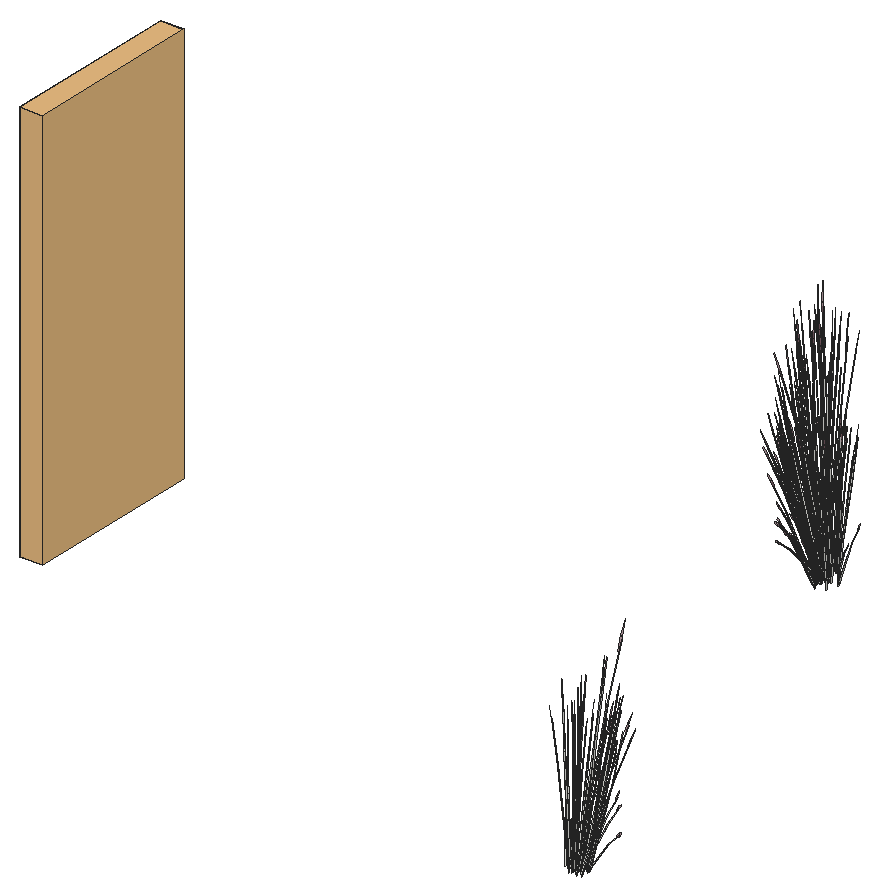
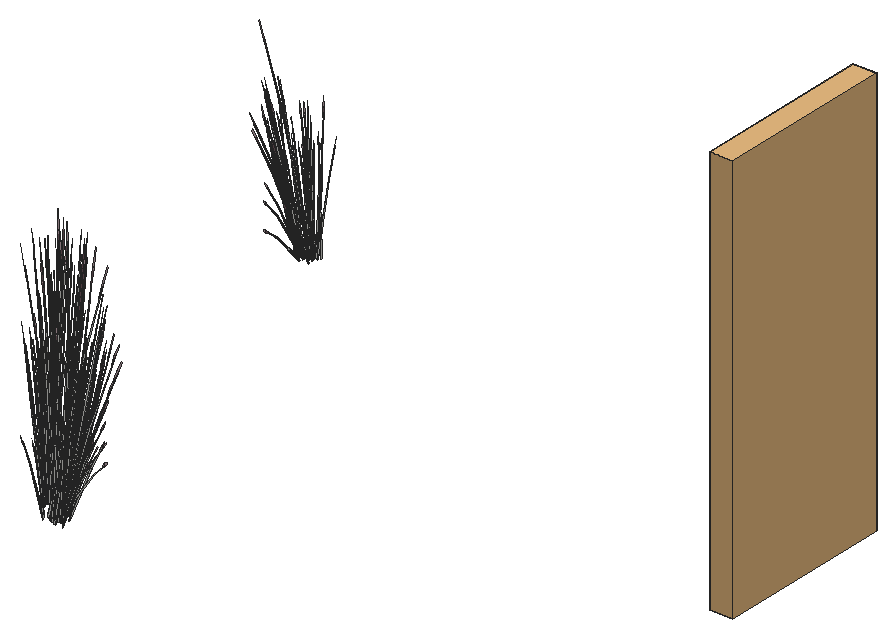
# SketchUp Ruby script. Lengths in inches.
U = 1.inch
M = Sketchup.active_model
def pt(a) = Geom::Point3d.new(a.map { |v| v * U })
def face(e, loops, mat)
  f = e.add_face(loops[0].map { |a| pt(a) })
  loops[1..].each { |l| e.add_face(l.map { |a| pt(a) }).erase! }
  f.material = f.back_material = mat if mat
  f
end
# faces: each face lists its corners as indices into pts; further lists are holes
def faces(e, pts, list, mat = nil) = list.each { |f| face(e, (f[0].is_a?(Array) ? f : [f]).map { |l| l.map { |i| pts[i] } }, mat) }
# xy, xz, yz: faces in a plane at the given z, y or x. An outline is a flat list of corners, or four numbers for a rectangle; further outlines are holes
def ring(l) = l.size == 4 ? [[l[0], l[1]], [l[2], l[1]], [l[2], l[3]], [l[0], l[3]]] : l.each_slice(2).to_a
def flat(e, list, mat, &to3) = list.each { |f| face(e, (f[0].is_a?(Array) ? f : [f]).map { |l| ring(l).map { |u, v| to3.(u, v) } }, mat) }
def xy(e, z, list, mat = nil) = flat(e, list, mat) { |x, y| [x, y, z] }
def xz(e, y, list, mat = nil) = flat(e, list, mat) { |x, z| [x, y, z] }
def yz(e, x, list, mat = nil) = flat(e, list, mat) { |y, z| [x, y, z] }
def lines(e, pts, list) = list.each { |a, b| e.add_line(pt(pts[a]), pt(pts[b])) }
# prism: a flat outline (further loops are holes) pulled along v
def prism(e, loops, v, mat = nil)
  f = face(e, loops, mat); d = Geom::Vector3d.new(v.map { |x| x * U })
  f.pushpull(f.normal.samedirection?(d) ? d.length : -d.length)
end
def box(e, o, s, mat = nil) = prism(e, [[o, [o[0] + s[0], o[1], o[2]], [o[0] + s[0], o[1] + s[1], o[2]], [o[0], o[1] + s[1], o[2]]]], [0, 0, s[2]], mat)
def at(x, y, z, deg = 0) = Geom::Transformation.translation(pt([x, y, z])) * Geom::Transformation.rotation(ORIGIN, Z_AXIS, deg.degrees)
def axes(o, x, y, z) = Geom::Transformation.new([*x, 0, *y, 0, *z, 0, *pt(o).to_a, 1])
def part(name) = M.definitions.add(name)
# library, detail: a bought-in or finely detailed component or shape, given as its bounding box
def library(name, o, s) = part(name).tap { |d| box(d.entities, o, s) }
def detail(e, o, s) = box(e.add_group.entities, o, s)
def put(e, d, t, mat = nil) = e.add_instance(d, t).tap { |i| i.material = mat if mat }
def group(e, t, mat = nil) = e.add_group.tap { |g| g.transformation = t; g.material = mat if mat }.entities
root = M.entities
M.materials.add("LightPink_Translucent").color = [144, 107, 117]
M.materials["LightPink_Translucent"].alpha = 0.75
c1 = part("blade")
p = [[2.15,0.21,22],[0,0.17,0],[0.09,0.45,0],[2.18,0.31,22],[2.29,0.31,22],[0.38,0.45,0],
  [2.48,0.24,33],[2.49,0.24,33],[2.48,0.22,33]]
faces(c1.entities,p,[[0,1,2,3],[4,5,2,3],[6,3,4,7],[8,0,3,6]])
c2 = part("seeds")
p = [[0.3,-0.1,1.38],[-0.01,-0.03,1.59],[-0.01,-0.03,0.03],[0.14,-0.07,-0.07],[0.29,-0.03,3],[0.15,0.01,3.11]]
faces(c2.entities,p,[[0,1,2,3],[1,0,4,5]],"LightPink_Translucent")
c3 = part("blade with seeds")
put(c3.entities,c1,at(0,0,0))
put(c3.entities,c2,axes([2.4,0.25,30.99],[1.5799,-0.05474,1.17369],[-0.12525,1.92788,0.29478],[-0.07173,-0.02425,1.56792]))
c4 = library("porta+4",[0.2,-5.42,1.33],[46.55,4.72,83.21])
put(root,c3,axes([434.05,211.68,2.05],[0.08072,-0.00933,1.50452],[0.22141,-0.42869,-0.23794],[0.14358,0.05659,0.12066]))
put(root,c3,axes([430.82,211.26,2.07],[-0.09332,-0.50785,0.41282],[0.36608,-0.08814,0.34039],[-0.10789,0.11944,0.85423]))
put(root,c3,axes([430.75,211.16,2.07],[-0.25832,-0.23207,0.0553],[0.1504,-0.33047,0.43534],[-0.08282,0.10684,0.66383]))
put(root,c3,axes([430.87,210.55,1.33],[0.13056,-0.11672,1.47384],[0.10992,0.53933,0.11917],[-0.20497,0.12189,0.63005]))
put(root,c3,axes([431.05,211.09,2.34],[0.32754,-0.07886,0.30456],[0.08649,0.45081,-0.39319],[-0.09386,0.12109,0.75234]))
put(root,c3,axes([429.79,210.89,2.05],[0.04802,0.0148,1.5255],[0.14856,0.48754,-0.14414],[-0.0983,0.12796,0.26996]))
put(root,c3,axes([433.97,211.98,1.89],[0.2141,0.34548,-0.30456],[-0.24447,0.32704,0.39319],[0.12421,0.04976,0.75234]))
put(root,c3,axes([433.86,212.11,2.07],[-0.01895,0.4196,0.0553],[-0.28611,-0.0115,0.43534],[0.1096,0.04391,0.66383]))
put(root,c3,axes([430.78,211.36,1.89],[-0.32754,0.07886,-0.30456],[-0.08649,-0.45081,0.39319],[-0.09386,0.12109,0.75234]))
put(root,c3,axes([433.88,211.98,2.07],[-0.27746,0.36359,0.41282],[-0.23929,-0.38612,0.34039],[0.13017,0.06707,0.85423]))
put(root,c3,axes([430.31,212.37,2.86],[0.33205,0.14729,-0.05579],[-0.10214,0.45334,-0.25298],[-0.05431,0.06883,0.83441]))
put(root,c3,axes([433,212.4,2.34],[-0.05812,-0.44446,0.30456],[0.33222,-0.11736,-0.39319],[0.08923,0.12737,0.75234]))
put(root,c3,axes([433.2,211.09,1.33],[-0.13977,-0.09507,1.47384],[0.28925,-0.39884,0.11917],[0.18028,0.17992,0.63005]))
put(root,c3,axes([433.22,209.84,1.85],[-0.32515,-0.2867,1.18923],[0.34333,-0.44639,0.51312],[0.10491,0.26901,1.1495]))
put(root,c3,axes([430.88,211.05,2.33],[0.34807,0.30426,-0.10458],[-0.20053,0.44063,-0.58045],[-0.09834,0.15317,0.88199]))
put(root,c3,axes([432.97,212.625,2.33],[0.22423,-0.47232,-0.10458],[0.32472,0.27211,-0.58045],[0.11288,0.13344,0.88199]))
put(root,c3,axes([431.35,210.91,1.33],[0.09398,-0.16955,1.47384],[0.23731,0.45764,0.11917],[-0.16276,0.20841,0.63005]))
put(root,c3,axes([431.49,211.99,2.34],[0.2546,-0.29052,0.30456],[0.24101,0.33173,-0.39319],[-0.03667,0.16855,0.75234]))
put(root,c3,axes([432.68,213.02,2.05],[0.00111,-0.06681,1.5255],[0.32247,-0.29474,-0.14414],[0.11201,0.1052,0.26996]))
put(root,c3,axes([431.26,212.25,2.07],[-0.30922,-0.02571,0.0553],[0.00848,-0.38824,0.43534],[-0.03236,0.14872,0.66383]))
put(root,c3,axes([431.36,212.29,2.07],[-0.26795,-0.37649,0.41282],[0.28456,-0.3247,0.34039],[-0.04943,0.17664,0.85423]))
put(root,c3,axes([432.21,212.47,2.34],[0.11344,-0.42434,0.30456],[0.33096,0.12377,-0.39319],[0.03035,0.17085,0.75234]))
put(root,c3,axes([433.05,212.8,2.07],[-0.17102,0.35053,0.0553],[-0.24354,-0.20408,0.43534],[0.07874,0.11238,0.66383]))
put(root,c3,axes([432.65,213.98,2.86],[0.26003,-0.31656,-0.05579],[0.23826,0.3467,-0.25298],[0.01677,0.09824,0.83441]))
put(root,c3,axes([433.125,212.7,2.07],[-0.37426,0.12663,0.41282],[-0.06495,-0.49674,0.34039],[0.08802,0.1464,0.85423]))
put(root,c3,axes([431.28,211.33,1.33],[0.07006,-0.18966,1.47384],[0.29392,0.3925,0.11917],[-0.13259,0.24463,0.63005]))
put(root,c3,axes([432.1,212.85,2.07],[-0.27727,0.18753,0.0553],[-0.13571,-0.34197,0.43534],[0.02678,0.15075,0.66383]))
put(root,c3,axes([431.36,212.4,1.89],[-0.2546,0.29052,-0.30456],[-0.24101,-0.33173,0.39319],[-0.03667,0.16855,0.75234]))
put(root,c3,axes([430.48,212.32,2.05],[-0.00935,0.1092,1.50452],[0.26544,0.37987,-0.23794],[-0.06949,0.17964,0.12066]))
put(root,c3,axes([431.33,212.07,2.64],[0.41355,0.02734,-0.11608],[-0.0113,0.51765,-0.6443],[-0.02873,0.19937,0.97901]))
put(root,c3,axes([432.09,212.65,2.33],[0.36822,-0.25691,-0.10458],[0.18095,0.45596,-0.58045],[0.04858,0.19215,0.88199]))
put(root,c3,axes([432.2,212.82,2.35],[-0.37078,-0.14426,0.45823],[0.12679,-0.47426,0.37783],[0.02228,0.18651,0.9482]))
put(root,c3,axes([432.62,211.64,1.33],[-0.08601,-0.17716,1.47384],[0.39746,-0.14915,0.11917],[0.08983,0.27813,0.63005]))
put(root,c3,axes([432.24,212.91,1.89],[-0.11344,0.42434,-0.30456],[-0.33096,-0.12377,0.39319],[0.03035,0.17085,0.75234]))
put(root,c3,axes([430.45,213.43,2.05],[0.04269,-0.03331,1.5255],[0.35284,0.2216,-0.14414],[-0.00829,0.1845,0.26996]))
put(root,c3,axes([431.92,211.73,1.33],[-0.00921,-0.21179,1.47384],[0.39917,0.1405,0.11917],[-0.02469,0.30182,0.63005]))
put(root,c3,axes([432.01,213.67,2.05],[0.0477,0.08886,1.50452],[0.38493,0.03491,-0.23794],[0.03871,0.19596,0.12066]))
put(root,c4,axes([307.84,266.46,4.63],[0,-0.77596,0],[1,0,0],[0,0,0.99642]))
put(root,c3,axes([406.2,304.97,6.33],[0.08601,0.17716,1.47384],[-0.39746,0.14915,0.11917],[-0.08983,-0.27813,0.63005]))
put(root,c3,axes([406.86,303.79,7.05],[-0.05755,-0.07737,1.50452],[-0.38409,0.04905,-0.23794],[-0.0613,-0.18505,0.12066]))
put(root,c3,axes([407.75,304.71,5.23],[-0.10696,0.11169,1.22981],[-0.32033,-0.19549,-0.26449],[0.05938,-0.24312,0.52581]))
put(root,c3,axes([407.26,305.1,7.28],[-0.17959,-0.44867,-0.61099],[0.36969,-0.25004,0.07373],[-0.042,-0.21679,0.8643]))
put(root,c3,axes([406.09,304.5,5.23],[-0.02279,0.18051,1.22981],[-0.33311,0.15111,-0.26449],[-0.07787,-0.23331,0.52581]))
put(root,c3,axes([406.95,304.1,4.28],[-0.06312,0.01988,1.51654],[-0.34903,-0.22379,-0.23168],[0.00586,-0.18666,0.25832]))
put(root,c3,axes([408.01,305.54,7.28],[0.00979,-0.51041,-0.61099],[0.4123,0.03428,0.07373],[0.04351,-0.21623,0.8643]))
put(root,c3,axes([408.58,304.74,7.05],[-0.00363,-0.10982,1.50452],[-0.30678,-0.3174,-0.23794],[0.04743,-0.1924,0.12066]))
put(root,c3,axes([407.29,304.72,6.89],[0.11344,-0.42434,-0.30456],[0.33096,0.12377,0.39319],[-0.03035,-0.17085,0.75234]))
put(root,c3,axes([407.54,305.28,6.33],[-0.07006,0.18966,1.47384],[-0.29392,-0.3925,0.11917],[0.13259,-0.24463,0.63005]))
put(root,c3,axes([408.5,304.35,7.05],[-0.03821,0.04215,1.5255],[-0.37441,-0.1422,-0.14414],[-0.01355,-0.18393,0.26996]))
put(root,c3,axes([407.125,305.01,7.03],[-0.3699,-0.13833,-0.43945],[0.12679,-0.47426,-0.34039],[-0.03392,-0.19095,0.84085]))
put(root,c3,axes([407.35,303.82,5.38],[0.04827,0.32177,0.9878],[-0.26778,-0.17821,0.72577],[0.02882,-0.16476,0.21757]))
put(root,c3,axes([407.92,305.37,7.03],[-0.26937,-0.37076,-0.43945],[0.28456,-0.3247,-0.34039],[0.04099,-0.18838,0.84085]))
put(root,c3,axes([406.46,303.54,7.05],[-0.00702,0.06614,1.5255],[-0.34622,0.24004,-0.14414],[-0.10188,-0.1227,0.26996]))
put(root,c3,axes([406.39,304.71,7.38],[0.41917,-0.14183,0.46236],[0.07275,0.55635,0.38124],[-0.09858,-0.16397,0.95674]))
put(root,c3,axes([407.34,304.82,7.07],[0.37078,0.14426,0.41282],[-0.12679,0.47426,0.34039],[-0.02228,-0.18651,0.85423]))
put(root,c3,axes([407.44,304.99,7.33],[-0.36822,0.25691,-0.10458],[-0.18095,-0.45596,-0.58045],[-0.04858,-0.19215,0.88199]))
put(root,c3,axes([408.21,305.5625,7.33],[-0.41355,-0.02734,-0.10458],[0.0113,-0.51765,-0.58045],[0.02873,-0.19937,0.88199]))
put(root,c3,axes([408.18,305.23,6.89],[0.2546,-0.29052,-0.30456],[0.24101,0.33173,0.39319],[0.03667,-0.16855,0.75234]))
put(root,c3,axes([405.98,304.21,5.38],[0.19628,0.19205,0.9878],[-0.28586,0.11545,0.72577],[-0.06116,-0.1476,0.21757]))
put(root,c3,axes([407.43,304.78,7.07],[0.27727,-0.18753,0.0553],[0.13571,0.34197,0.43534],[-0.02678,-0.15075,0.66383]))
put(root,c3,axes([406.45,305.23,7.28],[-0.32086,-0.26671,-0.61099],[0.22803,-0.46737,0.07373],[-0.11625,-0.15925,0.8643]))
put(root,c3,axes([406.34,304.875,6.89],[-0.05812,-0.44446,-0.30456],[0.33222,-0.11736,0.39319],[-0.08923,-0.12737,0.75234]))
put(root,c3,axes([406.48,304.83,7.07],[0.17102,-0.35053,0.0553],[0.24354,0.20408,0.43534],[-0.07874,-0.11238,0.66383]))
put(root,c3,axes([405.82,304.79,4.28],[-0.03645,0.07269,1.51654],[-0.36835,0.15672,-0.23168],[-0.08898,-0.14257,0.25832]))
put(root,c3,axes([406.43,306.79,4.8],[-0.15453,-0.56584,-0.60058],[0.44514,-0.20379,-0.15763],[-0.01708,-0.19161,1.32568]))
put(root,c3,axes([405.625,305.52,6.33],[0.13977,0.09507,1.47384],[-0.28925,0.39884,0.11917],[-0.18028,-0.17992,0.63005]))
put(root,c3,axes([408.5,305.06,4.28],[-0.05632,-0.04347,1.51654],[-0.14467,-0.48565,-0.23168],[0.09759,-0.13179,0.25832]))
put(root,c3,axes([407.33,305.17,7.34],[-0.11344,0.42434,0.30456],[-0.33096,-0.12377,-0.39319],[-0.03035,-0.17085,0.75234]))
put(root,c3,axes([406.3,305.24,7.03],[-0.37131,0.13117,-0.43945],[-0.06495,-0.49674,-0.34039],[-0.09973,-0.14235,0.84085]))
put(root,c3,axes([408.18,305.34,7.07],[0.26795,0.37649,0.41282],[-0.28456,0.3247,0.34039],[0.04943,-0.17664,0.85423]))
put(root,c3,axes([406.5625,304.8,7.67],[-0.25113,0.52899,-0.11713],[-0.36369,-0.30476,-0.65011],[-0.12642,-0.14945,0.98783]))
put(root,c3,axes([408.28,305.38,7.07],[0.30922,0.02571,0.0553],[-0.00848,0.38824,0.43534],[0.03236,-0.14872,0.66383]))
put(root,c3,axes([408.04,305.64,7.34],[-0.2546,0.29052,0.30456],[-0.24101,-0.33173,-0.39319],[0.03667,-0.16855,0.75234]))
put(root,c3,axes([408.49,306.43,7.28],[0.19655,-0.43539,-0.61099],[0.34443,0.30942,0.07373],[0.11736,-0.15774,0.8643]))
put(root,c3,axes([406.37,305.16,5.04],[-0.23526,-0.55293,0],[0.3936,-0.30836,-0.44382],[0.08964,-0.07023,1.40792]))
put(root,c3,axes([408.48,306.22,7.03],[-0.09666,-0.50384,-0.43945],[0.36608,-0.08814,-0.34039],[0.10491,-0.13533,0.84085]))
put(root,c3,axes([406.89,304.49,4.83],[-0.26003,0.31656,-0.03348],[-0.23826,-0.3467,-0.15179],[-0.01677,-0.09824,0.50065]))
put(root,c3,axes([405.6,304.64,7.05],[-0.08096,-0.00389,1.50452],[-0.25776,0.38949,-0.23794],[-0.13753,-0.07958,0.12066]))
put(root,c3,axes([408.66,306.58,7.33],[-0.34807,-0.30426,-0.10458],[0.20053,-0.44063,-0.58045],[0.09834,-0.15317,0.88199]))
put(root,c3,axes([407.22,308.24,5.86],[0.32517,0.22251,1.30084],[-0.31856,0.47936,0.51441],[-0.14269,-0.28411,1.09053]))
put(root,c3,axes([406.54,305.24,7.34],[0.05812,0.44446,0.30456],[-0.33222,0.11736,-0.39319],[-0.08923,-0.12737,0.75234]))
put(root,c3,axes([405.52,306.71,4.74],[0,-0.5518,-0.427],[0.42099,0,0],[0,-0.12568,1.35453]))
put(root,c3,axes([406.6875,305.07,4.74],[0.35217,-0.2759,-0.427],[0.2105,0.49473,0],[0.08021,-0.06284,1.35453]))
put(root,c3,axes([408.78,306.03,5.23],[-0.13443,-0.01634,1.22981],[-0.13772,-0.43844,-0.26449],[0.16514,-0.12403,0.52581]))
put(root,c3,axes([405.54,305.53,7.38],[0.31075,-0.40722,0.46236],[0.268,0.43246,0.38124],[-0.14579,-0.07512,0.95674]))
put(root,c3,axes([409.51,306.45,7.05],[-0.04915,-0.00419,1.5255],[-0.20409,-0.44904,-0.14414],[0.08196,-0.14765,0.26996]))
put(root,c3,axes([407.11,306.2,4.77],[0.25345,-0.41475,-0.53624],[0.31485,0.37608,-0.14074],[0.10156,-0.10346,1.18365]))
put(root,c3,axes([408.93,305.22,5.38],[-0.12533,0.28089,0.9878],[-0.10773,-0.37739,0.72577],[0.10352,-0.09457,0.21757]))
put(root,c3,axes([408.75,306.28,6.89],[0.32754,-0.07886,-0.30456],[0.08649,0.45081,0.39319],[0.09386,-0.12109,0.75234]))
put(root,c3,axes([405.68,305.52,7.07],[0.01895,-0.4196,0.0553],[0.28611,0.0115,0.43534],[-0.1096,-0.04391,0.66383]))
put(root,c3,axes([406.66,306.93,4.9],[0.18257,-0.49721,-0.38476],[0.37935,0.23929,0.18517],[0,-0.11462,1.23533]))
put(root,c3,axes([405.57,305.66,6.89],[-0.2141,-0.34548,-0.30456],[0.24447,-0.32704,0.39319],[-0.12421,-0.04976,0.75234]))
put(root,c3,axes([406.83,306.69,5.29],[-0.04385,-0.62963,-0.25022],[0.45669,-0.03807,-0.43002],[0.08042,-0.08387,1.37348]))
put(root,c3,axes([405.7,306.72,4.74],[0.26266,-0.34428,-0.26641],[0.26266,0.34428,0.26641],[0,-0.11089,1.19518]))
put(root,c3,axes([405.59,305.07,4.83],[-0.10855,0.45057,-0.03348],[-0.33409,-0.1386,-0.15179],[-0.05073,-0.0737,0.50065]))
put(root,c3,axes([408.49,306.54,7.34],[-0.32754,0.07886,0.30456],[-0.08649,-0.45081,-0.39319],[0.09386,-0.12109,0.75234]))
put(root,c3,axes([406.62,307.34,5.29],[-0.42377,-0.26329,-0.25022],[0.20405,-0.55571,-0.43002],[-0.01332,-0.13644,1.37348]))
put(root,c3,axes([405.41,307.125,5.04],[-0.47052,0,0],[0,-0.61671,-0.44382],[0,-0.14046,1.40792]))
put(root,c3,axes([405.49,306.02,5.23],[0.07347,0.15363,1.22981],[-0.16929,0.41759,-0.26449],[-0.17383,-0.09981,0.52581]))
put(root,c3,axes([406.77,305.29,4.74],[0.35106,0.13653,-0.26641],[-0.08839,0.48081,0.26641],[0.07077,-0.05545,1.19518]))
put(root,c3,axes([405.8,305.89,7.28],[-0.37615,-0.01329,-0.61099],[0.02526,-0.55946,0.07373],[-0.15935,-0.05904,0.8643]))
put(root,c3,axes([408.78,306.47,7.07],[0.25832,0.23207,0.0553],[-0.1504,0.33047,0.43534],[0.08282,-0.10684,0.66383]))
put(root,c3,axes([408.71,306.375,7.07],[0.09332,0.50785,0.41282],[-0.36608,0.08814,0.34039],[0.10789,-0.11944,0.85423]))
put(root,c3,axes([409.7,306.99,7.05],[0.05222,-0.08405,1.50452],[-0.06683,-0.51557,-0.23794],[0.13101,-0.09775,0.12066]))
put(root,c3,axes([405.78,306.96,5],[-0.35001,0.46392,0.2645],[-0.35022,-0.45904,-0.31383],[-0.01222,-0.13174,1.41801]))
put(root,c3,axes([405.29,304.98,7.05],[0.0279,0.05507,1.5255],[-0.13448,0.49501,-0.14414],[-0.1362,0.00358,0.26996]))
put(root,c3,axes([406.89,307.18,5.09],[0.42398,0.26744,0.20696],[-0.20405,0.55571,0.43002],[0,-0.1281,1.38067]))
put(root,c3,axes([406.73,307.93,5.1],[0.09973,-0.65385,-0.20149],[0.47288,0.11397,0.44093],[-0.08263,-0.0903,1.34539]))
put(root,c3,axes([405.67,306,7.03],[-0.27323,0.36552,-0.43945],[-0.23929,-0.38612,-0.34039],[-0.13882,-0.05561,0.84085]))
put(root,c3,axes([405.875,305.84,7.34],[0.2141,0.34548,0.30456],[-0.24447,0.32704,-0.39319],[-0.12421,-0.04976,0.75234]))
put(root,c3,axes([405.06,306.48,5.38],[0.24023,-0.03948,0.9878],[-0.15239,0.3479,0.72577],[-0.11872,-0.05219,0.21757]))
put(root,c3,axes([406.75,306.81,5.34],[-0.40861,0.03406,0.38476],[-0.03695,-0.56543,-0.18517],[0.07315,-0.05731,1.23533]))
put(root,c3,axes([405.82,305.62,7.33],[-0.02015,0.56117,-0.10458],[-0.38148,-0.01534,-0.58045],[-0.14692,-0.03898,0.88199]))
put(root,c3,axes([405.7,307.22,5.13],[0,0.5518,0.427],[-0.42099,0,0],[0,-0.12568,1.35453]))
put(root,c3,axes([408.67,307.77,7.33],[-0.18933,-0.49965,-0.10458],[0.33602,-0.24554,-0.58045],[0.1416,-0.06592,0.88199]))
put(root,c3,axes([408.65,307.34,7.03],[0.10194,-0.50193,-0.43945],[0.34951,0.17204,-0.34039],[0.14072,-0.04602,0.84085]))
put(root,c3,axes([408.1,305.3,5.04],[0.23526,-0.55293,0],[0.3936,0.30836,-0.44382],[0.08964,0.07023,1.40792]))
put(root,c3,axes([405.33,306.39,6.33],[0.15608,-0.0125,1.47384],[-0.10354,0.54165,0.11917],[-0.22242,-0.0335,0.63005]))
put(root,c3,axes([406.69,307.66,4.9],[-0.22605,-0.46315,-0.38476],[0.34239,-0.32614,0.18517],[-0.07315,-0.05731,1.23533]))
put(root,c3,axes([406.74,307.01,5.03],[0.1636,0.61702,0.39349],[-0.46745,0.21456,0.15441],[0.00571,-0.11338,1.36617]))
put(root,c3,axes([409.03,307.48,4.7],[-0.24235,0.06622,1.21762],[-0.03858,-0.5271,0.0697],[0.16974,-0.07978,0.69287]))
put(root,c3,axes([409.47,307.02,4.94],[-0.23329,-0.35284,-0.05579],[0.2555,-0.3233,-0.25298],[0.0724,-0.02276,0.83441]))
put(root,c3,axes([406.66,307.5,5.34],[-0.18257,0.49721,0.38476],[-0.37935,-0.23929,-0.18517],[0,-0.11462,1.23533]))
put(root,c3,axes([407.33,307.0625,4.9],[0,-0.63847,0],[0.47052,0,0],[0,0,1.54332]))
put(root,c3,axes([407.9,305.59,5.13],[-0.35217,-0.2759,0.427],[0.2105,-0.49473,0],[0.08021,0.06284,1.35453]))
put(root,c3,axes([408.59,307.52,7.28],[0.33065,-0.2437,-0.61099],[0.18427,0.50165,0.07373],[0.15976,-0.05699,0.8643]))
put(root,c3,axes([406.49,307.84,4.77],[-0.39143,-0.09047,-0.53624],[0.0826,-0.55804,-0.14074],[-0.11681,-0.06762,1.18365]))
put(root,c3,axes([407.11,306.66,5.03],[-0.312,0.50076,0.39349],[-0.37066,-0.44204,0.15441],[0.07522,-0.04998,1.36617]))
put(root,c3,axes([407.45,307.56,4.98],[-0.35001,-0.47494,-0.05273],[0.35022,-0.47523,0],[-0.01222,-0.01659,1.50991]))
put(root,c3,axes([406.5625,305.84,5.13],[-0.1087,0.54839,0.15172],[-0.39778,-0.15519,0.30174],[0.06871,-0.00267,1.3795]))
put(root,c3,axes([408.54,307.62,7.34],[-0.31272,-0.15393,0.30456],[0.09121,-0.44909,-0.39319],[0.1259,-0.04118,0.75234]))
put(root,c3,axes([405.27,306.8,7.07],[0.10631,-0.50312,0.41282],[0.34951,0.17204,0.34039],[-0.13745,0.03024,0.85423]))
put(root,c3,axes([406.4,306.28,4.37],[-0.37038,0.22092,1.10879],[-0.11789,-0.63387,0.43083],[0.22743,0.01055,1.26112]))
put(root,c3,axes([407.39,306.44,5.25],[0.07259,-0.49245,0.12452],[0.35466,0.08548,-0.35559],[0.06454,0.05057,1.09]))
put(root,c3,axes([405.24,306.67,7.07],[-0.1382,-0.37624,0.0553],[0.25202,-0.18416,0.43534],[-0.11109,0.03633,0.66383]))
put(root,c3,axes([406.78,307.61,5.03],[0.4756,0.11626,0.39349],[-0.09679,0.6566,0.15441],[-0.0695,-0.0634,1.36617]))
put(root,c3,axes([409.29,307.14,4.28],[-0.01967,-0.08377,1.51654],[0.1364,-0.49004,-0.23168],[0.13759,-0.00705,0.25832]))
put(root,c3,axes([405.23,307.05,4.28],[0.00954,0.08696,1.51654],[-0.19238,0.45414,-0.23168],[-0.13665,-0.02289,0.25832]))
put(root,c3,axes([407.24,306.57,5.34],[-0.22605,-0.46315,0.38476],[0.34239,-0.32614,-0.18517],[0.07315,0.05731,1.23533]))
